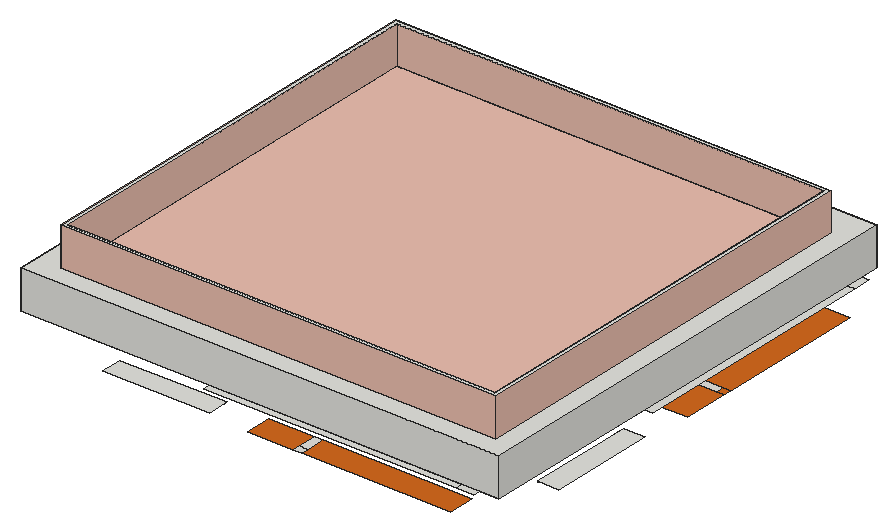
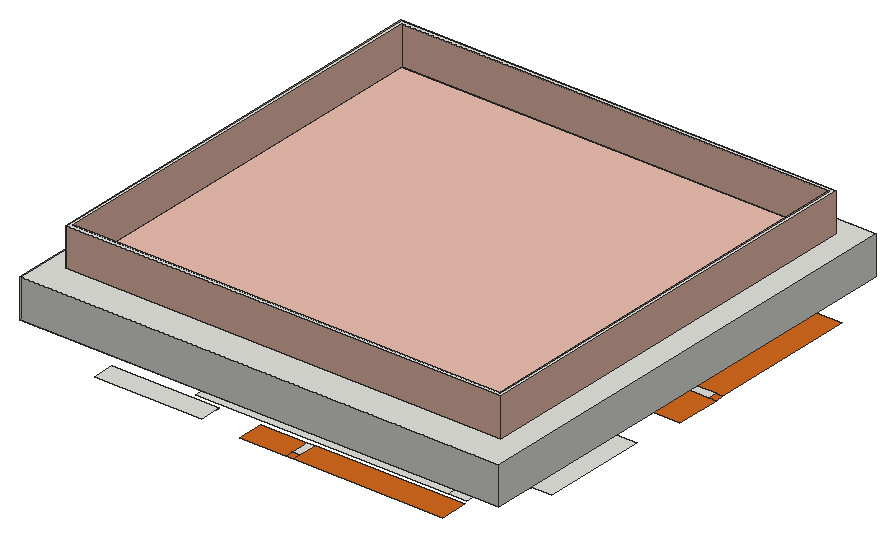
# SketchUp Ruby script. Lengths in inches.
U = 1.inch
M = Sketchup.active_model
def pt(a) = Geom::Point3d.new(a.map { |v| v * U })
def face(e, loops, mat)
  f = e.add_face(loops[0].map { |a| pt(a) })
  loops[1..].each { |l| e.add_face(l.map { |a| pt(a) }).erase! }
  f.material = f.back_material = mat if mat
  f
end
# faces: each face lists its corners as indices into pts; further lists are holes
def faces(e, pts, list, mat = nil) = list.each { |f| face(e, (f[0].is_a?(Array) ? f : [f]).map { |l| l.map { |i| pts[i] } }, mat) }
# xy, xz, yz: faces in a plane at the given z, y or x. An outline is a flat list of corners, or four numbers for a rectangle; further outlines are holes
def ring(l) = l.size == 4 ? [[l[0], l[1]], [l[2], l[1]], [l[2], l[3]], [l[0], l[3]]] : l.each_slice(2).to_a
def flat(e, list, mat, &to3) = list.each { |f| face(e, (f[0].is_a?(Array) ? f : [f]).map { |l| ring(l).map { |u, v| to3.(u, v) } }, mat) }
def xy(e, z, list, mat = nil) = flat(e, list, mat) { |x, y| [x, y, z] }
def xz(e, y, list, mat = nil) = flat(e, list, mat) { |x, z| [x, y, z] }
def yz(e, x, list, mat = nil) = flat(e, list, mat) { |y, z| [x, y, z] }
def lines(e, pts, list) = list.each { |a, b| e.add_line(pt(pts[a]), pt(pts[b])) }
# prism: a flat outline (further loops are holes) pulled along v
def prism(e, loops, v, mat = nil)
  f = face(e, loops, mat); d = Geom::Vector3d.new(v.map { |x| x * U })
  f.pushpull(f.normal.samedirection?(d) ? d.length : -d.length)
end
def box(e, o, s, mat = nil) = prism(e, [[o, [o[0] + s[0], o[1], o[2]], [o[0] + s[0], o[1] + s[1], o[2]], [o[0], o[1] + s[1], o[2]]]], [0, 0, s[2]], mat)
def at(x, y, z, deg = 0) = Geom::Transformation.translation(pt([x, y, z])) * Geom::Transformation.rotation(ORIGIN, Z_AXIS, deg.degrees)
def axes(o, x, y, z) = Geom::Transformation.new([*x, 0, *y, 0, *z, 0, *pt(o).to_a, 1])
def part(name) = M.definitions.add(name)
# library, detail: a bought-in or finely detailed component or shape, given as its bounding box
def library(name, o, s) = part(name).tap { |d| box(d.entities, o, s) }
def detail(e, o, s) = box(e.add_group.entities, o, s)
def put(e, d, t, mat = nil) = e.add_instance(d, t).tap { |i| i.material = mat if mat }
def group(e, t, mat = nil) = e.add_group.tap { |g| g.transformation = t; g.material = mat if mat }.entities
root = M.entities
M.materials.add("[0041_Chocolate]").color = [210, 105, 30]
M.materials.add("[0119_RosyBrown]").color = [234, 190, 174]
xy(root,1776.625,[[312.65,102.8125,473.9375,108.8125],[479.9375,102.8125,635.22,108.8125],[1476,277.47,1482,438.75],[1476,444.75,1482,600.03],[138,949.59,144,1104.875],
  [138,1110.875,144,1272.16],[984.78,1440.8125,1140.0625,1446.8125],[1146.0625,1440.8125,1307.35,1446.8125]])
xy(root,1782.625,[[306.65,36.8125,641.22,102.8125],[1482,271.47,1548,606.03],[72,943.59,138,1278.16],[978.78,1446.8125,1313.35,1512.8125]])
xy(root,1786.89,[[922.01,12.8125,948.52,36.8125],[922.01,36.8125,948.52,96.8125],[72,636.29,132,662.8],[1488,886.83,1548,913.33],[671.48,1452.8125,697.99,1512.8125]])
xy(root,1786.89,[[778.64,12.8125,922.01,96.8125],[948.52,12.8125,1414.89,96.8125],[48,169.92,132,636.29],[48,636.29,72,662.8],[48,662.8,132,806.17],
  [1488,743.45,1572,886.83],[1548,886.83,1572,913.33],[1488,913.33,1572,1379.7],[205.11,1452.8125,671.48,1536.8125],[697.99,1452.8125,841.36,1536.8125],
  [671.48,1512.8125,697.99,1536.8125]],"[0041_Chocolate]")
xy(root,1860,[[641.22,12.8125,1434.3125,12.8125,1434.3125,150.5,185.6875,150.5,185.6875,96.8125,246.65,96.8125,246.65,36.8125,641.22,36.8125],[1434.3125,12.8125,1488,150.5],[48,36.8125,1548,1512.8125],[48,96.8125,185.6875,150.5],[48,150.5,185.6875,150.5,185.6875,1399.125,132,1399.125,132,1338.16,72,1338.16,72,943.59,48,943.59],
  [1434.3125,150.5,1488,150.5,1488,211.46,1548,211.46,1548,606.03,1572,606.03,1572,1399.125,1434.3125,1399.125],[132,1399.125,185.6875,1536.8125],[185.6875,1399.125,1434.3125,1399.125,1434.3125,1452.8125,1373.35,1452.8125,1373.35,1512.8125,978.78,1512.8125,978.78,1536.8125,185.6875,1536.8125],[1434.3125,1399.125,1572,1452.8125]])
xy(root,1980,[[[48,36.8125,1548,1512.8125],[125.14,97.94,1487.02,1410.01]],[[125.14,97.94,1487.02,1410.01],[137.14,109.94,1475.02,1398.01]]])
xy(root,1980,[[137.14,109.94,1475.02,1398.01]],"[0119_RosyBrown]")
xy(root,2100,[[[125.14,97.94,1487.02,1410.01],[137.14,109.94,1475.02,1398.01]]])
xz(root,36.8125,[[48,1860,1548,1980]])
xz(root,97.94,[[125.14,1980,1487.02,2100]],"[0119_RosyBrown]")
xz(root,109.94,[[137.14,1980,1475.02,2100]],"[0119_RosyBrown]")
xz(root,1398.01,[[137.14,1980,1475.02,2100]],"[0119_RosyBrown]")
xz(root,1410.01,[[125.14,1980,1487.02,2100]],"[0119_RosyBrown]")
xz(root,1512.8125,[[48,1860,1548,1980]])
yz(root,48,[[36.8125,1860,1512.8125,1980]])
yz(root,125.14,[[97.94,1980,1410.01,2100]],"[0119_RosyBrown]")
yz(root,137.14,[[109.94,1980,1398.01,2100]],"[0119_RosyBrown]")
yz(root,1475.02,[[109.94,1980,1398.01,2100]],"[0119_RosyBrown]")
yz(root,1487.02,[[97.94,1980,1410.01,2100]],"[0119_RosyBrown]")
yz(root,1548,[[36.8125,1860,1512.8125,1980]])
